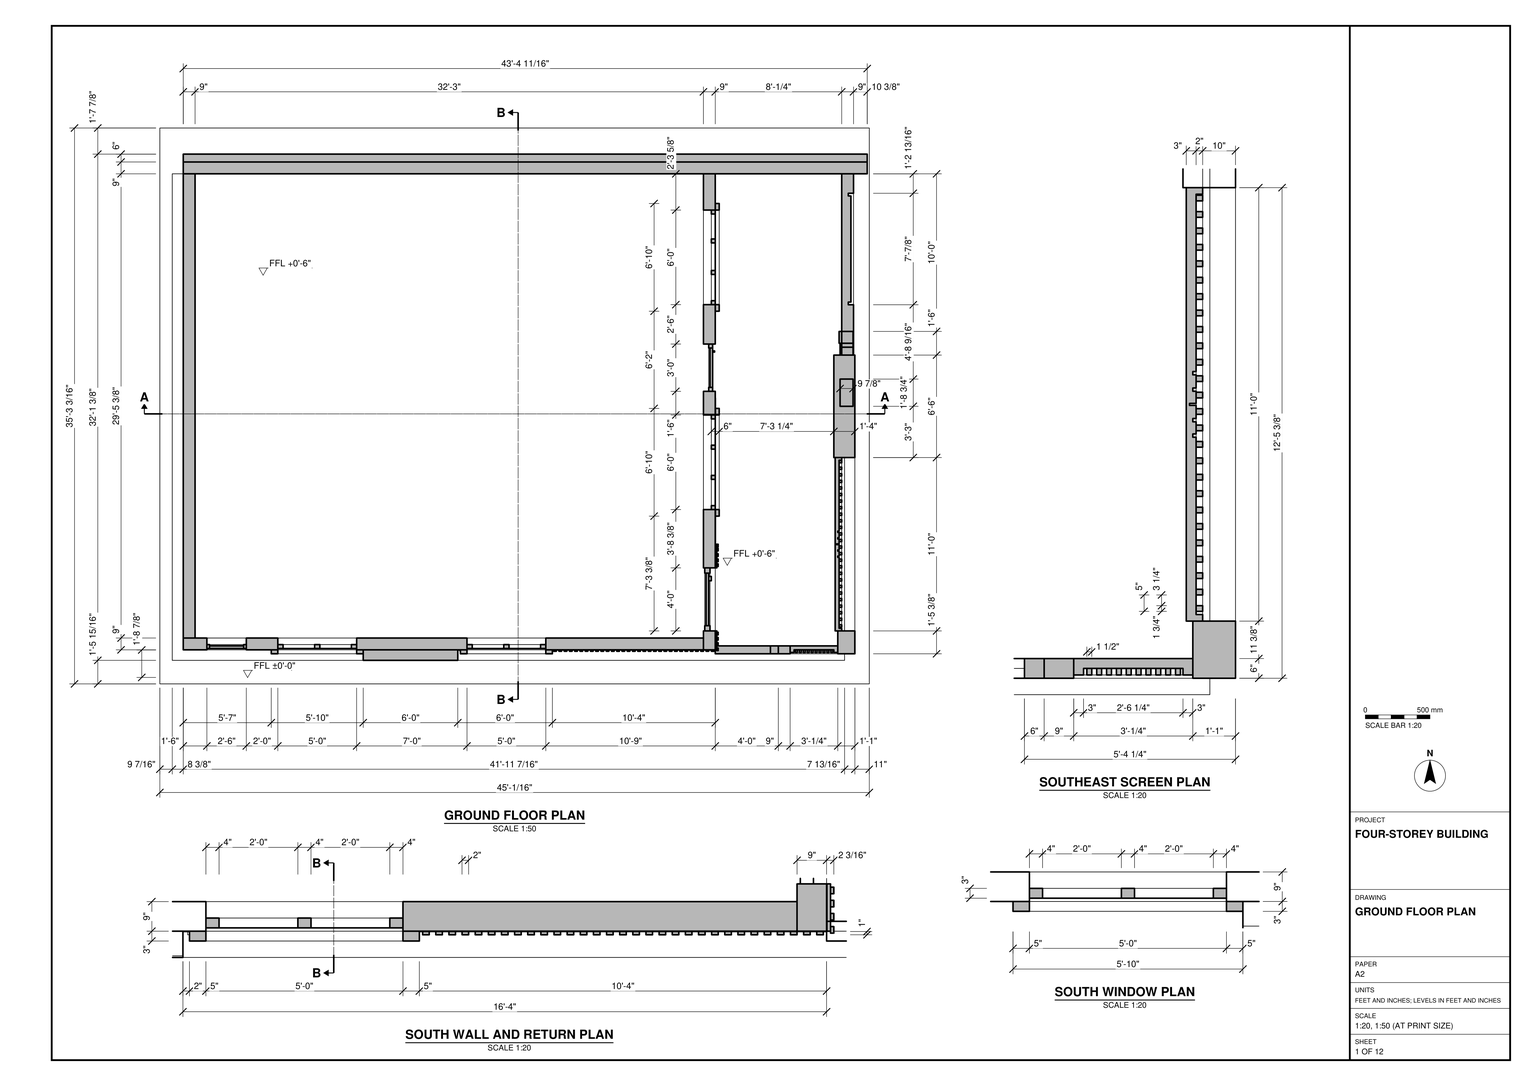
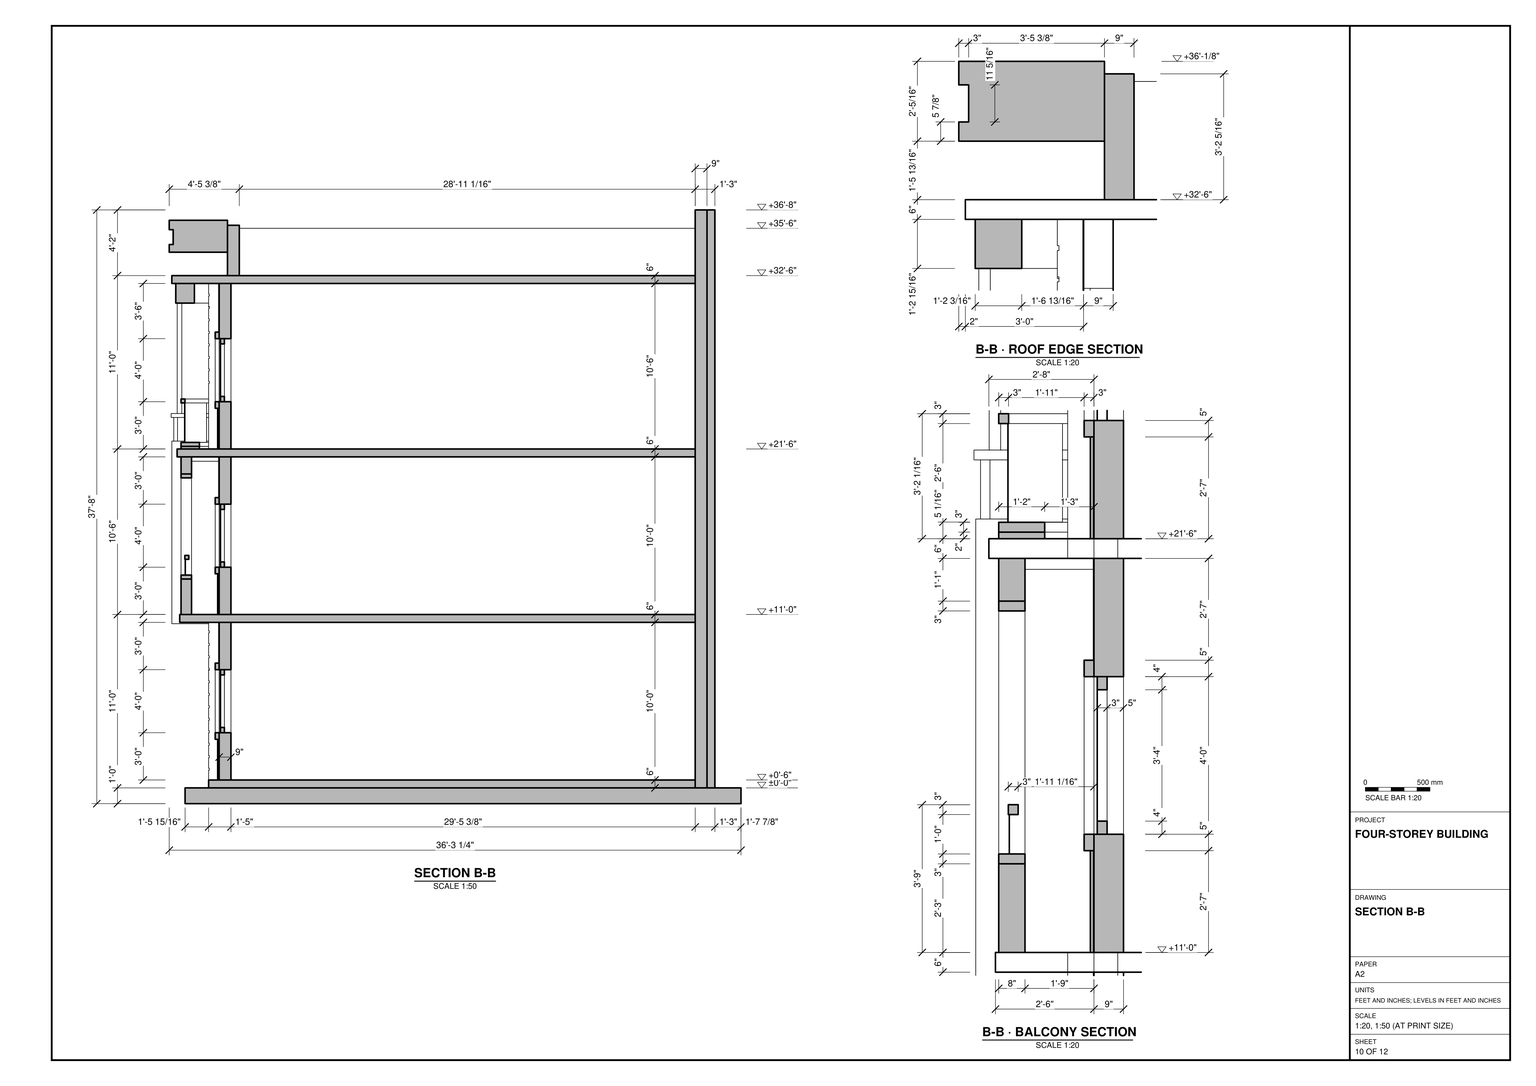
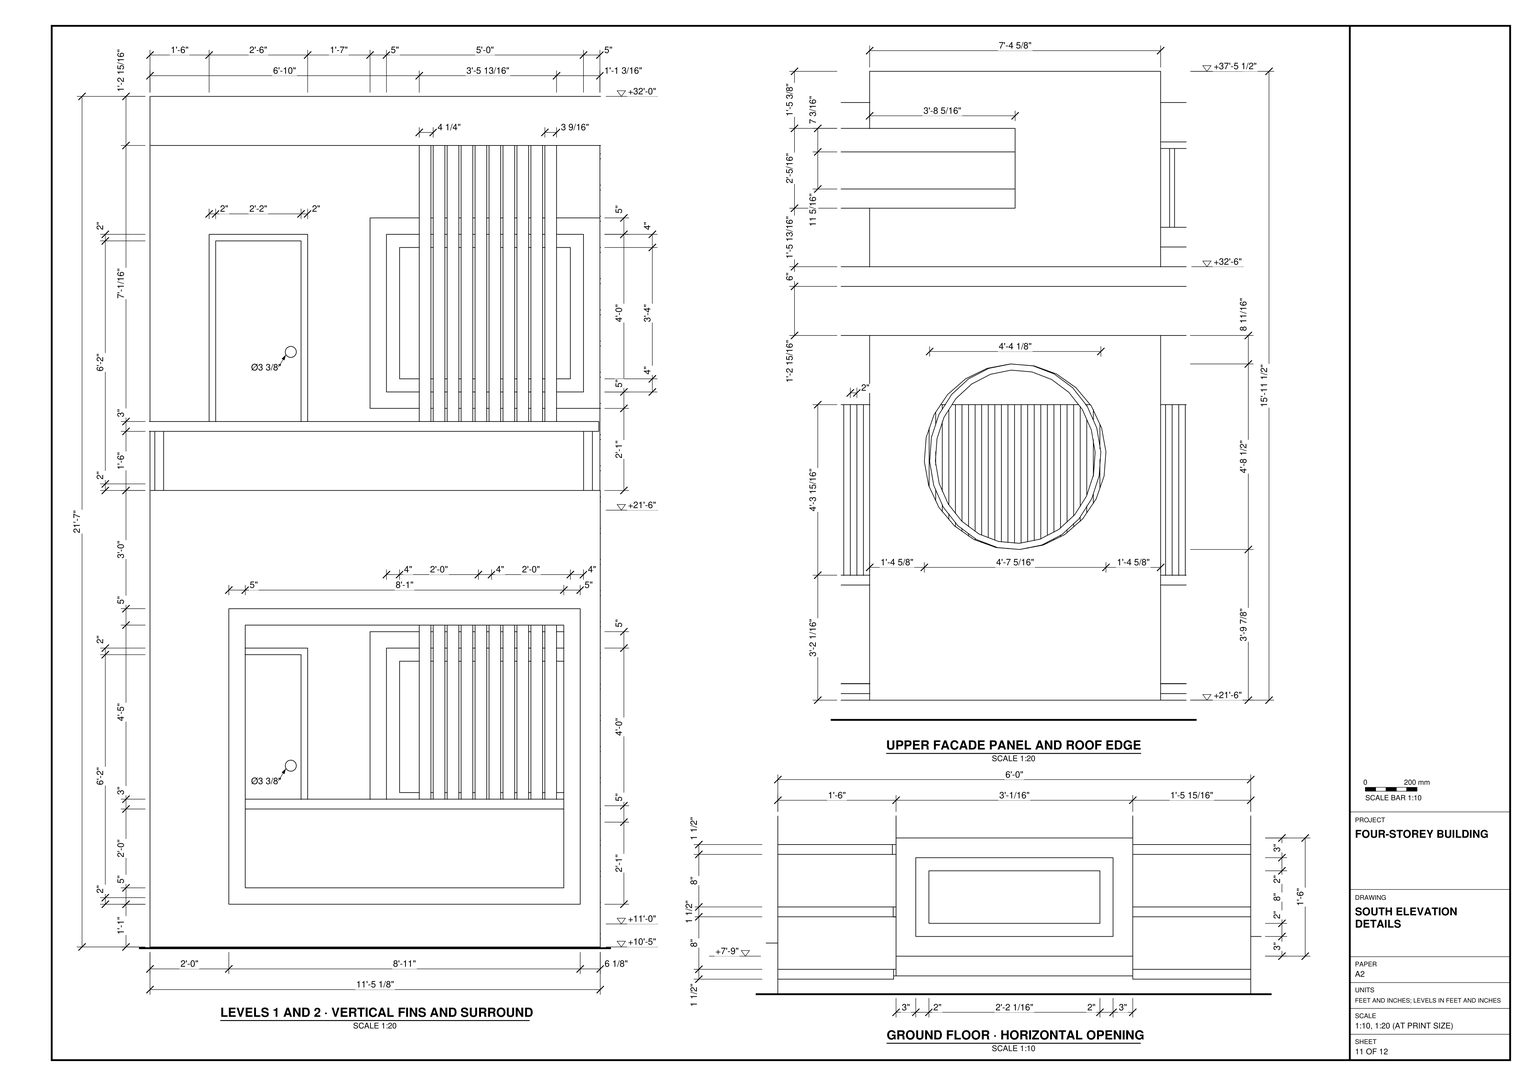
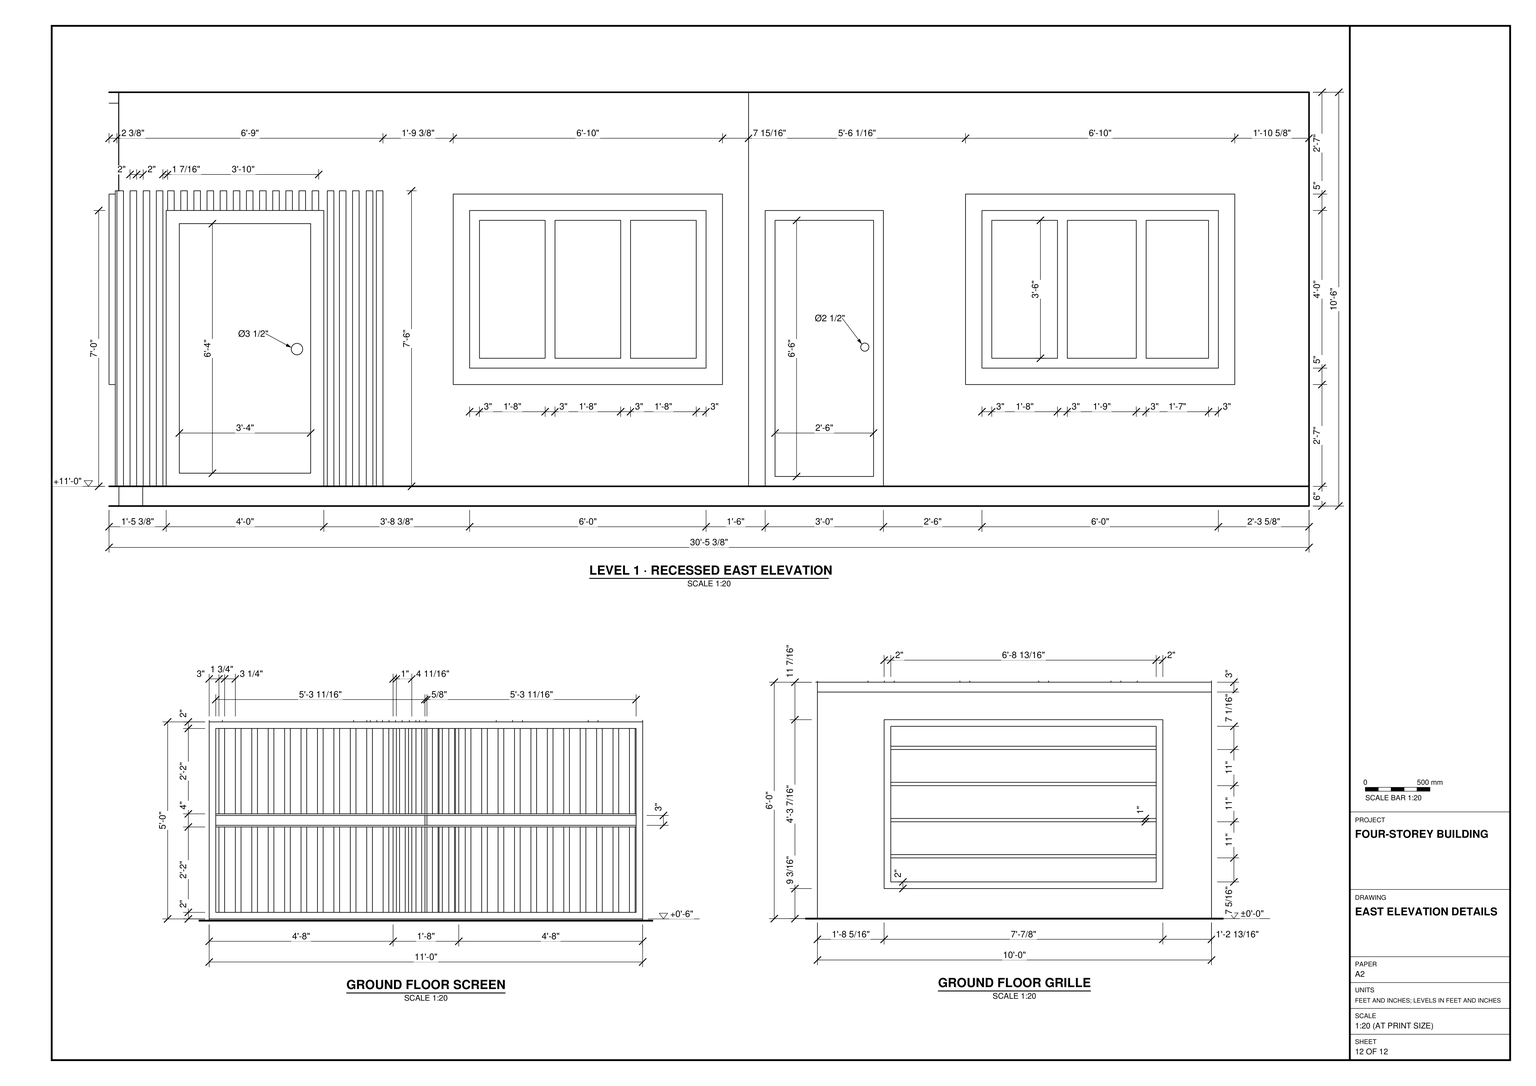
Build the building shown in task_files/diagram_01.pdf in SketchUp. Work in feet and inches. The overall model is 45'-5 1/2" along x, 36'-3 1/4" along y and 38'-5 1/2" high. Use ±0'-0" as the ground-floor reference, with upper floors at +11'-0" and +21'-6" and the roof slab at +32'-6". Distinguish the raised ground-floor finish from the reference level.

Follow the plans for the wall thicknesses, doorways and window openings. Keep the large ground-floor space and the narrow bay along its east side in their drawn relationship. Use the sections to set the slab edges, balcony projections, guards and parapets. On the south facade, model the framed windows, the small horizontal opening and the return at the southeast screen. Reproduce the different arrangements of surrounds and vertical fins on the two upper floors, including the circular opening in the upper facade panel. Use the sheets to place any stairs, built-in joinery and main furniture where shown.

Keep walls, slabs, roof elements and each furniture or joinery piece in separate groups or components, and use components for repeated parts. Decor and loose items may be any suitable library components. Save one SketchUp model as output_files/building_with_balconies_and_a_screened_south_facade.skp.

# SketchUp Ruby script. Lengths in inches.
U = 1.inch
M = Sketchup.active_model
def pt(a) = Geom::Point3d.new(a.map { |v| v * U })
def face(e, loops, mat)
  f = e.add_face(loops[0].map { |a| pt(a) })
  loops[1..].each { |l| e.add_face(l.map { |a| pt(a) }).erase! }
  f.material = f.back_material = mat if mat
  f
end
# faces: each face lists its corners as indices into pts; further lists are holes
def faces(e, pts, list, mat = nil) = list.each { |f| face(e, (f[0].is_a?(Array) ? f : [f]).map { |l| l.map { |i| pts[i] } }, mat) }
# xy, xz, yz: faces in a plane at the given z, y or x. An outline is a flat list of corners, or four numbers for a rectangle; further outlines are holes
def ring(l) = l.size == 4 ? [[l[0], l[1]], [l[2], l[1]], [l[2], l[3]], [l[0], l[3]]] : l.each_slice(2).to_a
def flat(e, list, mat, &to3) = list.each { |f| face(e, (f[0].is_a?(Array) ? f : [f]).map { |l| ring(l).map { |u, v| to3.(u, v) } }, mat) }
def xy(e, z, list, mat = nil) = flat(e, list, mat) { |x, y| [x, y, z] }
def xz(e, y, list, mat = nil) = flat(e, list, mat) { |x, z| [x, y, z] }
def yz(e, x, list, mat = nil) = flat(e, list, mat) { |y, z| [x, y, z] }
def lines(e, pts, list) = list.each { |a, b| e.add_line(pt(pts[a]), pt(pts[b])) }
# prism: a flat outline (further loops are holes) pulled along v
def prism(e, loops, v, mat = nil)
  f = face(e, loops, mat); d = Geom::Vector3d.new(v.map { |x| x * U })
  f.pushpull(f.normal.samedirection?(d) ? d.length : -d.length)
end
def box(e, o, s, mat = nil) = prism(e, [[o, [o[0] + s[0], o[1], o[2]], [o[0] + s[0], o[1] + s[1], o[2]], [o[0], o[1] + s[1], o[2]]]], [0, 0, s[2]], mat)
def at(x, y, z, deg = 0) = Geom::Transformation.translation(pt([x, y, z])) * Geom::Transformation.rotation(ORIGIN, Z_AXIS, deg.degrees)
def axes(o, x, y, z) = Geom::Transformation.new([*x, 0, *y, 0, *z, 0, *pt(o).to_a, 1])
def part(name) = M.definitions.add(name)
# library, detail: a bought-in or finely detailed component or shape, given as its bounding box
def library(name, o, s) = part(name).tap { |d| box(d.entities, o, s) }
def detail(e, o, s) = box(e.add_group.entities, o, s)
def put(e, d, t, mat = nil) = e.add_instance(d, t).tap { |i| i.material = mat if mat }
def group(e, t, mat = nil) = e.add_group.tap { |g| g.transformation = t; g.material = mat if mat }.entities
root = M.entities
M.materials.add("[Color E08]").color = [73, 73, 0]
M.materials.add("[Color M00]").color = [255, 255, 255]
M.materials.add("[Color M02]").color = [198, 198, 198]
M.materials.add("[Color M06]").color = [86, 86, 86]
M.materials.add("[Color M07]").color = [58, 58, 58]
M.materials.add("[Color M09]").color = [0, 0, 0]
M.materials.add("[Granite Brown]").color = [145, 119, 104]
M.materials.add("[Tile Grey]").color = [145, 145, 145]
M.materials.add("[Tile Mosaic Multi]1").color = [135, 103, 96]
M.materials.add("[Translucent Glass Gray]").color = [128, 128, 128]
M.materials["[Translucent Glass Gray]"].alpha = 0.5
M.materials.add("[Wood Floor Dark]").color = [153, 94, 42]
M.materials.add("[Wood Floor Light]").color = [219, 206, 168]
M.materials.add("[Wood Floor]").color = [117, 79, 46]
M.materials.add("[Wood Floor]1").color = [155, 105, 61]
M.materials.add("[Wood Veneer 01]").color = [86, 50, 26]
M.materials.add("[Wood Veneer 01]1").color = [120, 70, 37]
c1 = library("Group\#7",[0,0,0],[9,120,72])
c2 = library("Group\#18",[0,0,0],[5,132,60])
c3 = part("Group\#19")
prism(c3.entities,[[[4,0,84],[4,0,0],[4,48,0],[4,48,84]],[[4,44,4],[4,4,4],[4,4,80],[4,44,80]]],[-4,0,0])
c4 = part("Group\#20")
box(c4.entities,[0,0,0],[2,40,76])
c5 = part("Group\#26")
prism(c5.entities,[[[0,36,0],[0,0,0],[0,0,84],[0,36,84]],[[0,3,3],[0,33,3],[0,33,81],[0,3,81]]],[3,0,0])
c6 = part("Group\#27")
box(c6.entities,[0,0,0],[2,30,78])
c7 = part("Group\#28")
prism(c7.entities,[[[0,0,58],[0,82,58],[0,82,0],[0,0,0]],[[0,77,53],[0,5,53],[0,5,5],[0,77,5]]],[3,0,0])
c8 = part("Group\#29")
prism(c8.entities,[[[0,0,48],[0,72,48],[0,72,0],[0,0,0]],[[0,47,3],[0,47,45],[0,26,45],[0,26,3]],[[0,23,45],[0,3,45],[0,3,3],[0,23,3]],[[0,50,3],[0,69,3],[0,69,45],[0,50,45]]],[3,0,0])
c9 = part("Group\#30")
yz(c9.entities,0,[[0,0,19,42]])
c10 = part("Group\#31")
yz(c10.entities,0,[[0,0,21,42]])
c11 = part("Group\#32")
yz(c11.entities,0,[[0,0,20,42]])
c12 = library("Group\#33",[0,0,0],[1.5,2.5,2.5])
c13 = library("Group\#34",[0,0,0],[2,3.5,3.5])
c14 = part("Group\#96")
prism(c14.entities,[[[254.73,9,0],[-93.27,9,0],[-141.27,9,0],[-141.27,9,120],[254.73,9,120]],[[-9.27,9,84],[-69.27,9,84],[-69.27,9,36],[-9.27,9,36]],[[74.73,9,84],[74.73,9,36],[134.73,9,36],[134.73,9,84]],[[-123.27,9,6],[-93.27,9,6],[-93.27,9,84],[-123.27,9,84]],[[49.77,9,105],[13.73,9,105],[13.73,9,87],[49.77,9,87]]],[0,-9,0])
c15 = part("Group\#36")
prism(c15.entities,[[[0,0,48],[0,0,0],[60,0,0],[60,0,48]],[[28,0,44],[28,0,4],[4,0,4],[4,0,44]],[[32,0,44],[56,0,44],[56,0,4],[32,0,4]]],[0,3,0])
c16 = part("Group\#37")
xz(c16.entities,0,[[0,0,24,40]])
c17 = part("Group\#38")
xz(c17.entities,0,[[0,0,24,40]])
c18 = part("Group\#42")
prism(c18.entities,[[[0,0,48],[0,0,0],[60,0,0],[60,0,48]],[[28,0,44],[28,0,4],[4,0,4],[4,0,44]],[[32,0,44],[56,0,44],[56,0,4],[32,0,4]]],[0,3,0])
c19 = part("Group\#43")
xz(c19.entities,0,[[0,0,24,40]])
c20 = part("Group\#44")
prism(c20.entities,[[[30,0,78],[0,0,78],[0,0,0],[30,0,0]],[[28,0,2],[2,0,2],[2,0,76],[28,0,76]]],[0,3,0])
c21 = part("Group\#45")
box(c21.entities,[0,0,0],[26,2,74])
c22 = part("Group\#47")
xz(c22.entities,0,[[0,0,24,40]])
c23 = part("Group\#48")
prism(c23.entities,[[[70,3,0],[0,3,0],[0,3,58],[70,3,58]],[[65,3,5],[65,3,53],[5,3,53],[5,3,5]]],[0,-3,0])
c24 = part("Group\#51")
prism(c24.entities,[[[70,0,58],[0,0,58],[0,0,0],[70,0,0]],[[5,0,5],[5,0,53],[65,0,53],[65,0,5]]],[0,3,0])
c25 = library("Group\#63",[0,0,0],[36.27,5,60])
c26 = part("Group\#64")
prism(c26.entities,[[[-72,0.1,90],[0,0.1,90],[124,0.1,90],[124,0.1,0],[-72,0.1,0]],[[0,0.1,31],[0,0.1,89],[-70,0.1,89],[-70,0.1,31]]],[0,-0.1,0])
c27 = part("Group\#66")
box(c27.entities,[0,0,0],[2,1,90])
c28 = part("Group\#67")
put(c28.entities,c27,at(72,0,0))
put(c28.entities,c27,at(8,0,0))
put(c28.entities,c27,at(4,0,0))
put(c28.entities,c27,at(40,0,0))
put(c28.entities,c27,at(12,0,0))
put(c28.entities,c27,at(32,0,0))
put(c28.entities,c27,at(20,0,0))
put(c28.entities,c27,at(64,0,0))
put(c28.entities,c27,at(76,0,0))
put(c28.entities,c27,at(80,0,0))
put(c28.entities,c27,at(84,0,0))
put(c28.entities,c27,at(116,0,0))
put(c28.entities,c27,at(16,0,0))
put(c28.entities,c27,at(112,0,0))
put(c28.entities,c27,at(0,0,0))
put(c28.entities,c27,at(48,0,0))
put(c28.entities,c27,at(96,0,0))
put(c28.entities,c27,at(56,0,0))
put(c28.entities,c27,at(108,0,0))
put(c28.entities,c27,at(60,0,0))
put(c28.entities,c27,at(92,0,0))
put(c28.entities,c27,at(68,0,0))
put(c28.entities,c27,at(100,0,0))
put(c28.entities,c27,at(104,0,0))
put(c28.entities,c27,at(120,0,0))
put(c28.entities,c27,at(88,0,0))
put(c28.entities,c27,at(36,0,0))
put(c28.entities,c27,at(44,0,0))
put(c28.entities,c27,at(28,0,0))
put(c28.entities,c27,at(52,0,0))
put(c28.entities,c27,at(24,0,0))
c29 = part("Group\#68")
box(c29.entities,[0,0,0],[2,1,31])
c30 = part("Group\#69")
put(c30.entities,c29,at(56,0,0))
put(c30.entities,c29,at(12,0,0))
put(c30.entities,c29,at(36,0,0))
put(c30.entities,c29,at(40,0,0))
put(c30.entities,c29,at(48,0,0))
put(c30.entities,c29,at(20,0,0))
put(c30.entities,c29,at(4,0,0))
put(c30.entities,c29,at(24,0,0))
put(c30.entities,c29,at(28,0,0))
put(c30.entities,c29,at(0,0,0))
put(c30.entities,c29,at(16,0,0))
put(c30.entities,c29,at(52,0,0))
put(c30.entities,c29,at(60,0,0))
put(c30.entities,c29,at(64,0,0))
put(c30.entities,c29,at(68,0,0))
put(c30.entities,c29,at(32,0,0))
put(c30.entities,c29,at(44,0,0))
put(c30.entities,c29,at(8,0,0))
c31 = part("Group\#97")
xy(c31.entities,0,[[0,117.6,9,132],[0,180,9,314.4],[0,350.4,9,480]])
xy(c31.entities,36,[[0,224.4,9,296.4],[0,380.4,9,452.4]])
xy(c31.entities,84,[[0,132,9,180],[0,224.4,9,296.4],[0,314.4,9,350.4],[0,380.4,9,452.4]])
xy(c31.entities,120,[[0,117.6,9,480]])
xz(c31.entities,117.6,[[0,0,9,120]])
xz(c31.entities,132,[[0,0,9,84]])
xz(c31.entities,180,[[0,0,9,84]],"[Wood Veneer 01]1")
xz(c31.entities,224.4,[[0,36,9,84]])
xz(c31.entities,296.4,[[0,36,9,84]])
xz(c31.entities,314.4,[[0,0,9,84]])
xz(c31.entities,350.4,[[0,0,9,84]])
xz(c31.entities,380.4,[[0,36,9,84]])
xz(c31.entities,452.4,[[0,36,9,84]])
xz(c31.entities,480,[[0,0,9,120]])
yz(c31.entities,0,[[[117.6,0,117.6,120,480,120,480,0,350.4,0,350.4,84,314.4,84,314.4,0,180,0,180,84,132,84,132,0],[380.4,36,452.4,84],[224.4,36,296.4,84]]])
yz(c31.entities,9,[[[117.6,0,132,0,132,84,180,84,180,0,314.4,0,314.4,84,350.4,84,350.4,0,480,0,480,120,117.6,120],[224.4,36,296.4,84],[380.4,36,452.4,84]]])
c32 = part("Group\#35")
prism(c32.entities,[[[36.04,0,18],[0,0,18],[0,0,0],[36.04,0,0]],[[33.04,0,15],[33.04,0,3],[3,0,3],[3,0,15]]],[0,4,0])
c33 = part("Group\#39")
prism(c33.entities,[[[0,2,12],[30.04,2,12],[30.04,2,0],[0,2,0]],[[2,2,2],[28.04,2,2],[28.04,2,10],[2,2,10]]],[0,-2,0])
c34 = part("Group\#40")
xz(c34.entities,0,[[0,0,26.04,8]])
c35 = library("Group\#46",[0,0,0],[6,82,58])
c36 = library("Group\#49",[0,0,0],[3.375,1.5,3.375])
c37 = part("Group\#71")
box(c37.entities,[0,0,0],[1,2,6])
c38 = part("Group\#70")
box(c38.entities,[0,0,0],[1,2,90])
c39 = part("Group\#73")
box(c39.entities,[0,0,0],[1,2,90])
c40 = part("Group\#50")
g1 = group(c40.entities,at(0,15.4375,84),"[Wood Floor]1")
put(g1,c37,at(0,44,0))
put(g1,c37,at(0,20,0))
put(g1,c37,at(0,0,0))
put(g1,c37,at(0,12,0))
put(g1,c37,at(0,16,0))
put(g1,c37,at(0,8,0))
put(g1,c37,at(0,4,0))
put(g1,c37,at(0,32,0))
put(g1,c37,at(0,40,0))
put(g1,c37,at(0,24,0))
put(g1,c37,at(0,36,0))
put(g1,c37,at(0,28,0))
put(c40.entities,c38,at(0,71.75,0),"[Wood Floor]1")
put(c40.entities,c38,at(0,64.0625,0),"[Wood Floor]1")
put(c40.entities,c38,at(0,79,0),"[Wood Floor]1")
put(c40.entities,c38,at(0,67.75,0),"[Wood Floor]1")
put(c40.entities,c38,at(0,75.9375,0),"[Wood Floor]1")
g2 = group(c40.entities,at(0,0,0),"[Wood Floor]1")
put(g2,c39,at(0,12,0))
put(g2,c39,at(0,0,0))
put(g2,c39,at(0,8,0))
put(g2,c39,at(0,4,0))
c41 = part("Group\#98")
g3 = group(c41.entities,at(0,0,0))
xy(g3,0,[[196,0.1,196.1,14.5],[196,62.5,196.1,191.84]])
xy(g3,36,[[196,106.9,196.1,178.9]])
xy(g3,84,[[196,14.5,196.1,62.5],[196,106.9,196.1,178.9]])
xy(g3,90,[[0,0,196,0.1]])
xy(g3,120,[[0,0,196,0.1],[196,0.1,196.1,191.84]])
xz(g3,0,[[0,90,196,120]],"[Wood Floor Light]")
xz(g3,0.1,[[196,0,196.1,90],[0,90,196,120],[196,90,196.1,120]])
xz(g3,14.5,[[196,0,196.1,84]])
xz(g3,62.5,[[196,0,196.1,84]])
xz(g3,106.9,[[196,36,196.1,84]])
xz(g3,178.9,[[196,36,196.1,84]])
xz(g3,191.84,[[196,0,196.1,120]])
yz(g3,0,[[0,90,0.1,120]])
yz(g3,196,[[[0.1,0,0.1,120,191.84,120,191.84,0,62.5,0,62.5,84,14.5,84,14.5,0],[106.9,36,178.9,84]],[0,90,0.1,120]])
yz(g3,196.1,[[[0.1,0,14.5,0,14.5,84,62.5,84,62.5,0,191.84,0,191.84,120,0.1,120],[106.9,36,178.9,84]]],"[Wood Floor Light]")
p = [[196,62.5,0],[196,14.5,0]]
lines(g3,p,[[0,1]])
c42 = library("Group\#76",[0,-13,0],[72,21,378])
c43 = library("Group\#81",[0,0,0],[39,39,74])
c44 = library("Group\#95",[-2.97,0,9.18],[101.85,3.2,203.09])
c45 = part("Group\#102")
box(c45.entities,[0,0,0],[1.5,1.5,24])
c46 = part("Group\#108")
box(c46.entities,[0,0,0],[4.1875,3.5,241])
p = [[425.8125,221.8,107],[425.8125,139.8,107],[425.8125,139.8,49],[425.8125,221.8,49],[175.8125,38,234],[175.8125,38,246],
  [205.85,38,246],[205.85,38,234],[175.8125,38,360],[175.8125,38,372],[205.85,38,372],[205.85,38,360],
  [175.8125,38,108],[175.8125,38,120],[205.85,38,120],[205.85,38,108],[175.8125,36,246],[205.85,36,246],
  [205.85,36,234],[175.8125,36,234],[175.8125,36,360],[175.8125,36,372],[205.85,36,360],[205.85,36,372],
  [205.85,36,120],[205.85,36,108],[175.8125,36,120],[175.8125,36,108],[23.8125,8,144],[148.8125,8,144],
  [148.68,4.9,294],[148.68,4.9,297]]
lines(root,p,[[0,1],[1,2],[2,3],[3,0],[4,5],[5,6],[6,7],[7,4],[8,9],[9,10],[10,11],[11,8],
  [12,13],[13,14],[14,15],[15,12],[16,17],[18,19],[17,18],[20,21],[22,20],[23,22],[21,23],[24,25],
  [26,24],[27,26],[25,27],[5,16],[6,17],[4,19],[7,18],[8,20],[9,21],[11,22],[10,23],[14,24],
  [15,25],[13,26],[12,27],[28,29],[30,31]])
g4 = group(root,at(94.75,89.77,0))
box(g4,[-94.75,-77.6875,0],[540.08,423.1875,12])
g5 = group(root,at(159.08,-79.6,12))
box(g5,[-149.64,109.6,0],[511.83,370.4,6])
put(root,c1,at(519.08,280.4,12),"[Color M06]")
g6 = group(root,at(519.08,268.4,12))
box(g6,[0,0,0],[9,12,72])
g7 = group(root,at(519.08,262.4,12))
box(g7,[0,0,0],[9,6,72])
g8 = group(root,at(513.08,184.4,12),"[Granite Brown]")
xy(g8,0,[[6,0,16,78]])
xy(g8,6,[[0,0,6,78]])
xy(g8,69,[[0,0,16,78]])
xy(g8,72,[[0,0,16,78]])
xz(g8,0,[[6,0,16,0,16,69,0,69,0,6,6,6],[0,69,16,72]])
xz(g8,78,[[6,0,6,6,0,6,0,69,16,69,16,0],[0,69,16,72]])
yz(g8,0,[[0,6,78,69],[0,69,78,72]])
yz(g8,6,[[0,0,78,6]])
yz(g8,16,[[0,0,78,69],[0,69,78,72]])
put(root,c2,at(514.08,52.4,18))
put(root,c3,at(414.8125,52.4,18),"[Color M09]")
put(root,c4,at(415.8125,56.4,22),"[Wood Veneer 01]")
put(root,c5,at(417.8125,234.8,18),"[Color M09]")
put(root,c6,at(418.8125,237.8,21),"[Wood Veneer 01]")
put(root,c7,at(422.8125,295.8,49))
put(root,c8,at(419.8125,300.8,54),"[Color M09]")
put(root,c9,at(422.8125,350.8,57),"[Translucent Glass Gray]")
put(root,c10,at(422.8125,326.8,57),"[Translucent Glass Gray]")
put(root,c11,at(422.8125,303.8,57),"[Translucent Glass Gray]")
put(root,c12,at(420.8125,263.88,59.15))
put(root,c13,at(417.8125,90.48,58.05))
put(root,c14,at(159.08,38,18))
put(root,c15,at(233.8125,39,54),"[Color M09]")
put(root,c16,at(265.8125,39,58),"[Translucent Glass Gray]")
put(root,c17,at(237.8125,39,58),"[Translucent Glass Gray]")
put(root,c18,at(89.8125,39,54),"[Color M09]")
put(root,c19,at(121.8125,39,58),"[Translucent Glass Gray]")
put(root,c20,at(35.8125,39,24),"[Color M09]")
put(root,c21,at(37.8125,39,26),"[Wood Veneer 01]1")
put(root,c22,at(93.8125,39,58),"[Translucent Glass Gray]")
put(root,c23,at(84.8125,35,49),"[Color E08]")
put(root,c24,at(228.8125,35,49),"[Color M07]")
g9 = group(root,at(422.8125,35,12),"[Wood Floor Light]")
xy(g9,0,[[0,0,3,3],[3,0,7,3],[7,0,42,3]])
xy(g9,6,[[0,3,42,6]])
xy(g9,72,[[0,0,3,6],[3,0,7,6],[7,0,42,6]])
xz(g9,0,[[7,0,42,72]])
xz(g9,0,[[0,0,3,72]],"[Color M00]")
xz(g9,0,[[3,0,7,72]],"[Color M09]")
xz(g9,3,[[0,0,42,6]])
xz(g9,6,[[0,6,42,72]])
yz(g9,0,[[0,0,3,0,3,6,6,6,6,72,0,72]])
yz(g9,42,[[0,0,0,72,6,72,6,6,3,6,3,0]])
g10 = group(root,at(464.8125,35,12),"[Color M09]")
box(g10,[0,0,0],[6,6,72])
g11 = group(root,at(470.8125,35,12))
xy(g11,0,[[0,0,45.27,3]])
xy(g11,6,[[9,0,45.27,3],[0,3,9,6],[9,3,45.27,6]])
xy(g11,72,[[0,0,9,6]])
xz(g11,0,[[0,0,45.27,0,45.27,6,9,6,9,72,0,72]])
xz(g11,3,[[0,0,45.27,6]])
xz(g11,6,[[0,6,9,72]])
yz(g11,0,[[0,0,0,72,6,72,6,6,3,6,3,0]])
yz(g11,9,[[0,6,6,72]])
yz(g11,45.27,[[0,0,3,6]])
put(root,c25,at(479.8125,36,18))
put(root,c26,at(298.8125,37.9,18),"[Wood Floor]")
g12 = group(root,at(422.8125,38,18),"[Wood Floor]")
prism(g12,[[[1.2,0,0],[1.2,14.4,0],[1.2,14.4,84],[1.2,62.4,84],[1.2,62.4,0],[1.2,80.4,0],[1.2,80.4,90],[1.2,0,90]]],[-1.2,0,0])
put(root,c28,at(299.8125,36.9,18),"[Wood Floor]1")
put(root,c30,at(228.25,36.9,18),"[Wood Floor]1")
g13 = group(root,at(159.08,400.4,12))
xy(g13,0,[[-141.27,0,379.4,9]])
xy(g13,440,[[-141.27,0,379.4,9]])
xz(g13,0,[[291.31,15.03,338.56,368.16]],"[Color M00]")
xz(g13,0,[[[-141.27,0,379.4,440],[291.31,15.03,338.56,368.16]]],"[Wood Floor Light]")
xz(g13,9,[[-141.27,0,379.4,440]])
yz(g13,-141.27,[[0,0,9,440]])
yz(g13,379.4,[[0,0,9,440]],"[Wood Floor Light]")
g14 = group(root,at(159.08,409.4,12))
xy(g14,0,[[-141.27,0,379.4,6]])
xy(g14,440,[[-141.27,0,379.4,6]])
xz(g14,0,[[-141.27,0,379.4,440]])
xz(g14,6,[[-141.27,0,379.4,440]])
yz(g14,-141.27,[[0,0,6,440]])
yz(g14,379.4,[[0,0,6,440]],"[Color M09]")
put(root,c31,at(413.8125,-79.6,18))
put(root,c32,at(172.8125,36,105))
put(root,c33,at(175.8125,38,108),"[Color M09]")
put(root,c34,at(177.8125,38,110),"[Translucent Glass Gray]")
g15 = group(root,at(17.8125,38,138),"[Tile Mosaic Multi]1")
xy(g15,0,[[0,-30,0,362.4,520.67,362.4,520.67,378.4,527.67,378.4,527.67,-30,190.04,-30,190.04,-8,209,-8,209,0,137,0,137,-30]],"[Wood Floor Dark]")
xy(g15,6,[[0,-30,137,-30,137,0,209,0,209,-8,190.04,-8,190.04,-30,527.67,-30,527.67,378.4,520.67,378.4,520.67,362.4,0,362.4]])
xz(g15,-30,[[0,0,137,6],[190.04,0,527.67,6]])
xz(g15,-8,[[190.04,0,209,6]])
xz(g15,0,[[137,0,209,6]])
xz(g15,362.4,[[0,0,520.67,6]])
xz(g15,378.4,[[520.67,0,527.67,6]])
yz(g15,0,[[-30,0,362.4,6]],"[Color M00]")
yz(g15,137,[[-30,0,0,6]])
yz(g15,190.04,[[-30,0,-8,6]])
yz(g15,209,[[-8,0,0,6]])
yz(g15,520.67,[[362.4,0,378.4,6]])
yz(g15,527.67,[[-30,0,378.4,6]])
put(root,c35,at(419.8125,139.8,49))
put(root,c36,at(58.99,37.5,64.51))
put(root,c40,at(424.01,37.4,18))
put(root,c41,at(226.8125,37.9,18))
put(root,c34,at(177.8125,38,236),"[Translucent Glass Gray]")
g16 = group(root,at(17.8125,38,264),"[Tile Mosaic Multi]1")
xy(g16,0,[[190.04,-32,190.04,-8,209,-8,209,0,137,0,137,-30,0,-30,0,362.4,526.67,362.4,526.67,-32]],"[Wood Floor Dark]")
xy(g16,6,[[190.04,-32,526.67,-32,526.67,362.4,0,362.4,0,-30,137,-30,137,0,209,0,209,-8,190.04,-8]])
xz(g16,-32,[[190.04,0,526.67,6]])
xz(g16,-30,[[0,0,137,6]])
xz(g16,-8,[[190.04,0,209,6]])
xz(g16,0,[[137,0,209,6]])
xz(g16,362.4,[[0,0,526.67,6]])
yz(g16,0,[[-30,0,362.4,6]],"[Color M00]")
yz(g16,137,[[-30,0,0,6]])
yz(g16,190.04,[[-32,0,-8,6]])
yz(g16,209,[[-8,0,0,6]])
yz(g16,526.67,[[-32,0,362.4,6]])
put(root,c40,at(424.01,37.4,144))
put(root,c9,at(422.8125,350.8,183),"[Translucent Glass Gray]")
put(root,c35,at(419.8125,139.8,175))
put(root,c22,at(93.8125,39,184),"[Translucent Glass Gray]")
put(root,c7,at(422.8125,295.8,175))
put(root,c23,at(84.8125,35,175),"[Color E08]")
put(root,c8,at(419.8125,300.8,180),"[Color M09]")
put(root,c13,at(417.8125,90.48,184.05))
put(root,c19,at(121.8125,39,184),"[Translucent Glass Gray]")
put(root,c12,at(420.8125,263.88,185.15))
put(root,c20,at(35.8125,39,150),"[Color M09]")
put(root,c41,at(226.8125,37.9,144))
put(root,c36,at(58.99,37.5,190.51))
put(root,c18,at(89.8125,39,180),"[Color M09]")
put(root,c31,at(413.8125,-79.6,144))
put(root,c14,at(159.08,38,144))
put(root,c5,at(417.8125,234.8,144),"[Color M09]")
put(root,c10,at(422.8125,326.8,183),"[Translucent Glass Gray]")
put(root,c6,at(418.8125,237.8,147),"[Wood Veneer 01]")
put(root,c26,at(298.8125,37.9,144),"[Wood Floor]")
put(root,c4,at(415.8125,56.4,148),"[Wood Veneer 01]")
put(root,c30,at(228.25,36.9,144),"[Wood Floor]1")
put(root,c3,at(414.8125,52.4,144),"[Color M09]")
put(root,c24,at(228.8125,35,175),"[Color M07]")
put(root,c15,at(233.8125,39,180),"[Color M09]")
put(root,c11,at(422.8125,303.8,183),"[Translucent Glass Gray]")
put(root,c17,at(237.8125,39,184),"[Translucent Glass Gray]")
put(root,c16,at(265.8125,39,184),"[Translucent Glass Gray]")
put(root,c21,at(37.8125,39,152),"[Wood Veneer 01]1")
put(root,c28,at(299.8125,36.9,144),"[Wood Floor]1")
put(root,c32,at(172.8125,36,231))
put(root,c33,at(175.8125,38,234),"[Color M09]")
put(root,c21,at(37.8125,39,278),"[Wood Veneer 01]1")
put(root,c6,at(418.8125,237.8,273),"[Wood Veneer 01]")
put(root,c4,at(415.8125,56.4,274),"[Wood Veneer 01]")
put(root,c3,at(414.8125,52.4,270),"[Color M09]")
put(root,c11,at(422.8125,303.8,309),"[Translucent Glass Gray]")
put(root,c33,at(175.8125,38,360),"[Color M09]")
put(root,c32,at(172.8125,36,357))
put(root,c28,at(299.8125,36.9,270),"[Wood Floor]1")
g17 = group(root,at(159.08,38,270))
prism(g17,[[[254.73,9,0],[-93.27,9,0],[-141.27,9,0],[-141.27,9,126],[254.73,9,126]],[[-9.27,9,84],[-69.27,9,84],[-69.27,9,36],[-9.27,9,36]],[[74.73,9,84],[74.73,9,36],[134.73,9,36],[134.73,9,84]],[[-123.27,9,6],[-93.27,9,6],[-93.27,9,84],[-123.27,9,84]],[[49.77,9,105],[13.73,9,105],[13.73,9,87],[49.77,9,87]]],[0,-9,0])
put(root,c5,at(417.8125,234.8,270),"[Color M09]")
put(root,c26,at(298.8125,37.9,270),"[Wood Floor]")
put(root,c30,at(228.25,36.9,270),"[Wood Floor]1")
put(root,c24,at(228.8125,35,301),"[Color M07]")
put(root,c15,at(233.8125,39,306),"[Color M09]")
put(root,c16,at(265.8125,39,310),"[Translucent Glass Gray]")
put(root,c17,at(237.8125,39,310),"[Translucent Glass Gray]")
put(root,c19,at(121.8125,39,310),"[Translucent Glass Gray]")
put(root,c13,at(417.8125,90.48,310.05))
put(root,c36,at(58.99,37.5,316.51))
put(root,c34,at(177.8125,38,362),"[Translucent Glass Gray]")
g18 = group(root,at(17.8125,38,396),"[Color M06]")
xy(g18,0,[[0,-36,523.67,362.4]],"[Wood Floor Dark]")
xy(g18,6,[[0,-36,523.67,362.4]],"[Color M00]")
xz(g18,-36,[[0,0,523.67,6]])
xz(g18,362.4,[[0,0,523.67,6]])
yz(g18,0,[[-36,0,362.4,6]],"[Color M00]")
yz(g18,523.67,[[-36,0,362.4,6]])
put(root,c22,at(93.8125,39,310),"[Translucent Glass Gray]")
put(root,c40,at(424.01,37.4,270))
put(root,c7,at(422.8125,295.8,301))
put(root,c23,at(84.8125,35,301),"[Color E08]")
put(root,c9,at(422.8125,350.8,309),"[Translucent Glass Gray]")
put(root,c8,at(419.8125,300.8,306),"[Color M09]")
put(root,c35,at(419.8125,139.8,301))
put(root,c10,at(422.8125,326.8,309),"[Translucent Glass Gray]")
put(root,c12,at(420.8125,263.88,311.15))
put(root,c20,at(35.8125,39,276),"[Color M09]")
g19 = group(root,at(226.8125,37.9,270))
g20 = group(g19,at(0,0,0))
xy(g20,0,[[196,0.1,196.1,14.5],[196,62.5,196.1,191.84]])
xy(g20,36,[[196,106.9,196.1,178.9]])
xy(g20,84,[[196,14.5,196.1,62.5],[196,106.9,196.1,178.9]])
xy(g20,90,[[0,0,196,0.1]])
xy(g20,126,[[0,0,196,0.1],[196,0.1,196.1,191.84]])
xz(g20,0,[[0,90,196,126]],"[Wood Floor Light]")
xz(g20,0.1,[[196,0,196.1,90],[0,90,196,126],[196,90,196.1,126]])
xz(g20,14.5,[[196,0,196.1,84]])
xz(g20,62.5,[[196,0,196.1,84]])
xz(g20,106.9,[[196,36,196.1,84]])
xz(g20,178.9,[[196,36,196.1,84]])
xz(g20,191.84,[[196,0,196.1,126]])
yz(g20,0,[[0,90,0.1,126]])
yz(g20,196,[[[0.1,0,0.1,126,191.84,126,191.84,0,62.5,0,62.5,84,14.5,84,14.5,0],[106.9,36,178.9,84]],[0,90,0.1,126]])
yz(g20,196.1,[[[0.1,0,14.5,0,14.5,84,62.5,84,62.5,0,191.84,0,191.84,126,0.1,126],[106.9,36,178.9,84]]],"[Wood Floor Light]")
p = [[196,62.5,0],[196,14.5,0]]
lines(g20,p,[[0,1]])
put(root,c18,at(89.8125,39,306),"[Color M09]")
g21 = group(root,at(413.8125,-79.6,270))
xy(g21,0,[[0,117.6,9,132],[0,180,9,314.4],[0,350.4,9,480]])
xy(g21,36,[[0,224.4,9,296.4],[0,380.4,9,452.4]])
xy(g21,84,[[0,132,9,180],[0,224.4,9,296.4],[0,314.4,9,350.4],[0,380.4,9,452.4]])
xy(g21,126,[[0,117.6,9,480]])
xz(g21,117.6,[[0,0,9,126]])
xz(g21,132,[[0,0,9,84]])
xz(g21,180,[[0,0,9,84]],"[Wood Veneer 01]1")
xz(g21,224.4,[[0,36,9,84]])
xz(g21,296.4,[[0,36,9,84]])
xz(g21,314.4,[[0,0,9,84]])
xz(g21,350.4,[[0,0,9,84]])
xz(g21,380.4,[[0,36,9,84]])
xz(g21,452.4,[[0,36,9,84]])
xz(g21,480,[[0,0,9,126]])
yz(g21,0,[[[117.6,0,117.6,126,480,126,480,0,350.4,0,350.4,84,314.4,84,314.4,0,180,0,180,84,132,84,132,0],[380.4,36,452.4,84],[224.4,36,296.4,84]]])
yz(g21,9,[[[117.6,0,132,0,132,84,180,84,180,0,314.4,0,314.4,84,350.4,84,350.4,0,480,0,480,126,117.6,126],[224.4,36,296.4,84],[380.4,36,452.4,84]]])
put(root,c42,at(154.8125,30,18),"[Granite Brown]")
g22 = group(root,at(208.85,9,144),"[Tile Mosaic Multi]1")
xy(g22,0,[[0,0,0,8,329.63,8,329.63,406.4,335.63,406.4,335.63,0]])
xy(g22,27,[[17.96,0,335.63,0,335.63,373.36,329.63,373.36,329.63,8,17.96,8]])
xy(g22,30,[[17.96,0,335.63,0,335.63,373.36,329.63,373.36,329.63,8,17.96,8]],"[Color M09]")
xy(g22,104,[[17.96,0,17.96,8,329.63,8,329.63,373.36,335.63,373.36,335.63,0]],"[Color M09]")
xy(g22,107,[[17.96,0,17.96,8,329.63,8,329.63,373.36,335.63,373.36,335.63,0]])
xy(g22,120,[[0,0,335.63,0,335.63,406.4,329.63,406.4,329.63,8,0,8]])
xz(g22,0,[[0,0,335.63,0,335.63,27,17.96,27,17.96,107,335.63,107,335.63,120,0,120]])
xz(g22,0,[[17.96,27,335.63,30],[17.96,104,335.63,107]],"[Color M09]")
xz(g22,8,[[0,0,0,120,329.63,120,329.63,107,17.96,107,17.96,27,329.63,27,329.63,0],[17.96,27,329.63,30],[17.96,104,329.63,107]])
xz(g22,373.36,[[329.63,27,335.63,30],[329.63,104,335.63,107]])
xz(g22,373.36,[[329.63,30,335.63,104]],"[Color M09]")
xz(g22,406.4,[[329.63,0,335.63,120]])
yz(g22,0,[[0,0,8,120]])
yz(g22,17.96,[[0,27,8,30],[0,104,8,107]])
yz(g22,17.96,[[0,30,8,104]],"[Color M09]")
yz(g22,329.63,[[8,0,8,27,373.36,27,373.36,102,406.4,102,406.4,0],[8,27,373.36,30],[373.36,102,373.36,107,8,107,8,120,406.4,120,406.4,102],[8,104,373.36,107]])
yz(g22,335.63,[[0,0,406.4,0,406.4,120,0,120,0,107,373.36,107,373.36,27,0,27]])
yz(g22,335.63,[[0,27,373.36,30],[0,104,373.36,107]],"[Color M09]")
put(root,c43,at(503.8,11.92,174),"[Tile Grey]")
g23 = group(root,at(226.8125,11.92,186),"[Wood Veneer 01]")
box(g23,[0,0,0],[276.98,3,3])
g24 = group(root,at(226.8125,12.23,174),"[Translucent Glass Gray]")
xz(g24,0,[[0,0,276.98,12]])
g25 = group(root,at(539.8,50.92,186),"[Wood Veneer 01]")
box(g25,[0,0,0],[3,331.45,3])
g26 = group(root,at(541.3,50.92,174),"[Translucent Glass Gray]")
yz(g26,0,[[0,0,331.45,12]])
g27 = group(root,at(508.08,223.4,18))
xy(g27,0,[[9.75,0,19.625,20.73],[9.75,39,19.625,48],[9,48,19.625,57]])
xy(g27,347.3125,[[9.75,20.73,19.625,39]],"[Wood Floor Light]")
xy(g27,377.3125,[[9.75,0,19.625,48]])
xy(g27,377.3125,[[9,48,19.625,57]],"[Color M00]")
xz(g27,0,[[9.75,0,19.625,377.3125]])
xz(g27,20.73,[[9.75,0,19.625,347.3125]])
xz(g27,39,[[9.75,0,19.625,347.3125]],"[Wood Floor Light]")
xz(g27,48,[[9.75,0,19.625,377.3125]])
xz(g27,48,[[9,0,9.75,377.3125]],"[Color M06]")
xz(g27,57,[[9,0,19.625,377.3125]],"[Color M06]")
yz(g27,9,[[48,0,57,377.3125]],"[Color M06]")
yz(g27,9.75,[[0,0,0,377.3125,39,377.3125,39,347.3125,20.73,347.3125,20.73,0],[39,0,48,377.3125]])
yz(g27,19.625,[[0,0,20.73,0,20.73,347.3125,39,347.3125,39,0,48,0,48,377.3125,0,377.3125]])
yz(g27,19.625,[[48,0,57,377.3125]],"[Color M06]")
g28 = group(root,at(516.08,35,12))
xy(g28,0,[[0,0,13,17.4]])
xy(g28,126,[[0,0,13,17.4]])
xy(g28,382.125,[[0,0,13,17.4]])
xz(g28,0,[[0,126,13,382.125]])
xz(g28,0,[[0,0,13,126]],"[Color M06]")
xz(g28,17.4,[[0,126,13,382.125]])
xz(g28,17.4,[[0,0,13,126]],"[Color M06]")
yz(g28,0,[[0,126,17.4,382.125]])
yz(g28,0,[[0,0,17.4,126]],"[Color M06]")
yz(g28,13,[[0,126,17.4,382.125]])
yz(g28,13,[[0,0,17.4,126]],"[Color M06]")
g29 = group(root,at(226.8125,17,144))
box(g29,[0,0,0],[0.1875,20.9,116.67])
g30 = group(root,at(208.85,9,275.0625))
g31 = group(g30,at(0,0,30),"[Wood Veneer 01]")
prism(g31,[[[312.63,391.4,0],[315.63,391.4,0],[315.63,0,0],[0,0,0],[0,21,0],[3,21,0],[3,3,0],[312.63,3,0]]],[0,0,3])
g32 = group(g30,at(0,2.8125,0),"[Translucent Glass Gray]")
xz(g32,0,[[0,0,315.63,30]])
yz(g32,0,[[0,0,16.61,30]])
yz(g32,315.63,[[0,0,26,30]])
g33 = group(g30,at(315.63,43.4,0),"[Translucent Glass Gray]")
yz(g33,0,[[0,0,348,30]])
put(root,c44,axes([316.27,6,261.34],[0.87,0,0],[0,2.61,0],[0,0,0.94294]))
g34 = group(root,at(208.98,9,270))
xy(g34,0,[[0,0,0,21,12.14,21,12.14,14,324.51,14,324.51,0],[312.51,14,324.51,391.4]])
xy(g34,2,[[0,0,324.51,0,324.51,391.4,312.51,391.4,312.51,14,12.14,14,12.14,21,0,21]])
xy(g34,5,[[0,0,324.51,0,324.51,391.4,312.51,391.4,312.51,14,12.14,14,12.14,21,0,21]],"[Granite Brown]")
xz(g34,0,[[0,0,324.51,2]])
xz(g34,0,[[0,2,324.51,5]],"[Granite Brown]")
xz(g34,14,[[12.14,0,312.51,2],[12.14,2,312.51,5]])
xz(g34,21,[[0,0,12.14,2],[0,2,12.14,5]])
xz(g34,391.4,[[312.51,0,324.51,2],[312.51,2,324.51,5]])
yz(g34,0,[[0,0,21,2]])
yz(g34,0,[[0,2,21,5]],"[Granite Brown]")
yz(g34,12.14,[[14,0,21,2],[14,2,21,5]])
yz(g34,312.51,[[14,0,391.4,2],[14,2,391.4,5]])
yz(g34,324.51,[[0,0,391.4,2]])
yz(g34,324.51,[[0,2,391.4,5]],"[Granite Brown]")
g35 = group(root,at(17.8125,5,381.06),"[Color M06]")
prism(g35,[[[0,0,0],[0,33,0],[10.6,33,0],[10.6,14.17,0],[510.93,14.17,0],[510.93,395.4,0],[520.67,395.4,0],[520.67,0,0]]],[0,0,14.94])
g36 = group(root,at(313.69,14.36,402))
xy(g36,0,[[9,0,216.43,6],[216.43,0,222.43,386.04]])
xy(g36,6,[[9,-0.875,216.43,0],[216.43,-0.875,223.3,0],[9,0,216.43,6],[216.43,0,222.43,386.04],[222.43,0,223.3,386.04]])
xy(g36,12,[[9,-0.875,223.3,-0.875,223.3,386.04,216.43,386.04,216.43,6,9,6]],"[Wood Veneer 01]")
xz(g36,-0.875,[[9,6,223.3,12]],"[Wood Veneer 01]")
xz(g36,0,[[9,0,222.43,6]])
xz(g36,6,[[9,0,216.43,6],[9,6,216.43,12]])
xz(g36,386.04,[[216.43,0,222.43,6],[216.43,6,223.3,12]])
yz(g36,9,[[0,0,6,6],[-0.875,6,6,12]])
yz(g36,216.43,[[6,0,386.04,6],[6,6,386.04,12]])
yz(g36,222.43,[[0,0,386.04,6]])
yz(g36,223.3,[[-0.875,6,386.04,12]],"[Wood Veneer 01]")
put(root,c45,at(531.04,16.36,414))
put(root,c45,at(522.04,16.36,414))
put(root,c45,at(513.04,16.36,414))
put(root,c45,at(504.04,16.36,414))
put(root,c45,at(495.04,16.36,414))
put(root,c45,at(486.04,16.36,414))
put(root,c45,at(477.04,16.36,414))
put(root,c45,at(468.04,16.36,414))
put(root,c45,at(459.04,16.36,414))
put(root,c45,at(450.04,16.36,414))
put(root,c45,at(441.04,16.36,414))
put(root,c45,at(432.04,16.36,414))
put(root,c45,at(423.04,16.36,414))
put(root,c45,at(414.04,16.36,414))
put(root,c45,at(405.04,16.36,414))
put(root,c45,at(531.04,25.36,414))
put(root,c45,at(531.04,34.36,414))
put(root,c45,at(531.04,43.36,414))
put(root,c45,at(531.04,52.36,414))
put(root,c45,at(531.04,61.36,414))
put(root,c45,at(531.04,70.36,414))
put(root,c45,at(531.04,79.36,414))
put(root,c45,at(531.04,88.36,414))
put(root,c45,at(531.04,97.36,414))
put(root,c45,at(531.04,106.36,414))
put(root,c45,at(531.04,115.36,414))
put(root,c45,at(531.04,124.36,414))
put(root,c45,at(531.04,133.36,414))
put(root,c45,at(531.04,142.36,414))
put(root,c45,at(531.04,151.36,414))
put(root,c45,at(531.04,160.36,414))
put(root,c45,at(531.04,169.36,414))
put(root,c45,at(531.04,178.36,414))
put(root,c45,at(531.04,187.36,414))
put(root,c45,at(531.04,196.36,414))
put(root,c45,at(531.04,205.36,414))
put(root,c45,at(531.04,214.36,414))
put(root,c45,at(531.04,223.36,414))
put(root,c45,at(531.04,232.36,414))
put(root,c45,at(531.04,241.36,414))
put(root,c45,at(531.04,250.36,414))
put(root,c45,at(531.04,259.36,414))
put(root,c45,at(531.04,268.36,414))
put(root,c45,at(531.04,277.36,414))
put(root,c45,at(531.04,286.36,414))
put(root,c45,at(531.04,295.36,414))
put(root,c45,at(531.04,304.36,414))
put(root,c45,at(531.04,313.36,414))
put(root,c45,at(531.04,322.36,414))
put(root,c45,at(531.04,331.36,414))
put(root,c45,at(531.04,340.36,414))
put(root,c45,at(531.04,349.36,414))
put(root,c45,at(531.04,358.36,414))
put(root,c45,at(531.04,367.36,414))
put(root,c45,at(531.04,376.36,414))
put(root,c45,at(531.04,385.36,414))
put(root,c45,at(531.04,394.36,414))
put(root,c45,at(396.04,16.36,414))
g37 = group(root,at(17.8125,20.36,402))
box(g37,[0,33,0],[9,347.04,36])
g38 = group(root,at(17.8125,8,144))
box(g38,[0,0,0],[9,30,120])
g39 = group(root,at(17.8125,2,138),"[Wood Floor Light]")
xy(g39,-1,[[0,0,0,6,131,6,131,43.25,137.1,43.25,137.1,0]])
xy(g39,12,[[24,0,131,6]])
xy(g39,102,[[24,0,131,6]])
xy(g39,138,[[0,0,137.1,0,137.1,43.25,131,43.25,131,6,0,6]])
xz(g39,0,[[[0,-1,137.1,138],[24,12,131,102]]])
xz(g39,6,[[0,-1,0,138,131,138,131,102,24,102,24,12,131,12,131,-1]])
xz(g39,43.25,[[131,-1,137.1,138]])
yz(g39,0,[[0,-1,6,138]])
yz(g39,24,[[0,12,6,102]])
yz(g39,131,[[6,-1,43.25,12],[0,12,43.25,102],[6,102,43.25,138]])
yz(g39,137.1,[[0,-1,43.25,138]])
g40 = group(root,at(41.8125,2,150),"[Color M09]")
prism(g40,[[[0,0,90],[0,0,0],[107,0,0],[107,0,90]],[[102,0,5],[5,0,5],[5,0,85],[102,0,85]]],[0,9,0])
g41 = group(root,at(99.8,6.09,155))
put(g41,c46,axes([38.25,0,0],[0.85,0,0],[0,1,0],[0,0,1]))
put(g41,c46,axes([12.75,0,0],[0.85,0,0],[0,1,0],[0,0,1]))
put(g41,c46,axes([21.25,0,0],[0.85,0,0],[0,1,0],[0,0,1]))
put(g41,c46,axes([8.5,0,0],[0.85,0,0],[0,1,0],[0,0,1]))
put(g41,c46,axes([17,0,0],[0.85,0,0],[0,1,0],[0,0,1]))
put(g41,c46,axes([34,0,0],[0.85,0,0],[0,1,0],[0,0,1]))
put(g41,c46,axes([0,0,0],[0.85,0,0],[0,1,0],[0,0,1]))
put(g41,c46,axes([25.5,0,0],[0.85,0,0],[0,1,0],[0,0,1]))
put(g41,c46,axes([4.25,0,0],[0.85,0,0],[0,1,0],[0,0,1]))
put(g41,c46,axes([29.75,0,0],[0.85,0,0],[0,1,0],[0,0,1]))
g42 = group(root,at(19.28,3.46,276),"[Color M09]")
box(g42,[0,0,0],[2.6875,2.875,18])
g43 = group(root,at(149.84,3.46,276),"[Color M09]")
box(g43,[0,0,0],[2.6875,2.875,18])
g44 = group(root,at(19.28,35.125,276),"[Color M09]")
box(g44,[0,0,0],[2.6875,2.875,18])
g45 = group(root,at(149.84,33.96,276),"[Color M09]")
box(g45,[0,0,0],[2.6875,2.875,18])
g46 = group(root,at(152.53,6.34,276),"[Translucent Glass Gray]")
yz(g46,0,[[0,0,27.625,18]])
g47 = group(root,at(21.96,3.46,276),"[Translucent Glass Gray]")
xz(g47,0,[[0,0,127.875,18]])
g48 = group(root,at(17.8125,6.34,270),"[Color M00]")
xy(g48,0,[[0,1.66,6,31.66]])
xy(g48,6,[[0,1.66,6,31.66]])
xz(g48,1.66,[[0,0,6,6]])
xz(g48,31.66,[[0,0,6,6]])
yz(g48,0,[[1.66,0,31.66,6]])
yz(g48,1.46,[[0,6,28.79,24]],"[Translucent Glass Gray]")
yz(g48,6,[[1.66,0,31.66,6]])
g49 = group(root,at(17.28,35.125,294),"[Wood Veneer 01]")
prism(g49,[[[0,2.875,0],[4.6875,2.875,0],[4.6875,-30.23,0],[131.41,-30.23,0],[131.41,2.875,0],[137.1875,2.875,0],[137.1875,-33.66,0],[0,-33.66,0]]],[0,0,3])
g50 = group(root,at(46.8125,3,155))
xy(g50,24,[[0,0,97,3.67]])
xy(g50,27,[[0,0,97,3.67]])
xz(g50,0,[[0,0,97,24]],"[Translucent Glass Gray]")
xz(g50,0,[[0,24,97,27]],"[Wood Veneer 01]")
xz(g50,3.67,[[0,24,97,27]])
yz(g50,0,[[0,24,3.67,27]])
yz(g50,97,[[0,24,3.67,27]])
g51 = group(root,at(89.9375,0,422.3125),"[Color M02]")
xy(g51,-2.5,[[0,0,0,44.36,223.76,44.36,223.76,6,268.06,6,268.06,0]])
xy(g51,3.35,[[0,0,268.06,3]])
xy(g51,14.65,[[0,0,268.06,3]])
xy(g51,21.8125,[[0,0,268.06,0,268.06,6,223.76,6,223.76,44.36,0,44.36]])
xz(g51,0,[[0,-2.5,268.06,3.35],[0,14.65,268.06,21.8125]])
xz(g51,3,[[0,3.35,268.06,14.65]])
xz(g51,6,[[223.76,-2.5,268.06,21.8125]])
xz(g51,44.36,[[0,-2.5,223.76,21.8125]])
yz(g51,0,[[0,-2.5,0,3.35,3,3.35,3,14.65,0,14.65,0,21.8125,44.36,21.8125,44.36,-2.5]])
yz(g51,223.76,[[6,-2.5,44.36,21.8125]])
yz(g51,268.06,[[0,-2.5,6,-2.5,6,21.8125,0,21.8125,0,14.65,3,14.65,3,3.35,0,3.35]])
g52 = group(root,at(26.8125,44.36,402))
box(g52,[-9,0,0],[295.88,9,38.3125])
g53 = group(root,at(313.69,14.36,402))
box(g53,[0,0,0],[9,39,38.3125])
g54 = group(root,at(396.04,16.36,438),"[Color M09]")
xy(g54,0,[[0,0,0,1.5,135,1.5,135,384.04,137,384.04,137,0]])
xy(g54,2,[[0,0,137,0,137,384.04,135,384.04,135,1.5,0,1.5]])
xz(g54,0,[[0,0,137,2]],"[Color M09]")
xz(g54,1.5,[[0,0,135,2]])
xz(g54,384.04,[[135,0,137,2]])
yz(g54,0,[[0,0,1.5,2]])
yz(g54,135,[[1.5,0,384.04,2]])
yz(g54,137,[[0,0,384.04,2]])
g55 = group(root,at(516.08,52.4,12))
box(g55,[0,0,0],[13,132,2.875])
g56 = group(root,at(17.8125,47,18))
box(g56,[0,0,0],[9,353.4,120])
g57 = group(root,at(17.8125,47,144))
box(g57,[0,0,0],[9,353.4,120])
g58 = group(root,at(17.8125,47,270))
box(g58,[0,0,0],[9,353.4,126])
